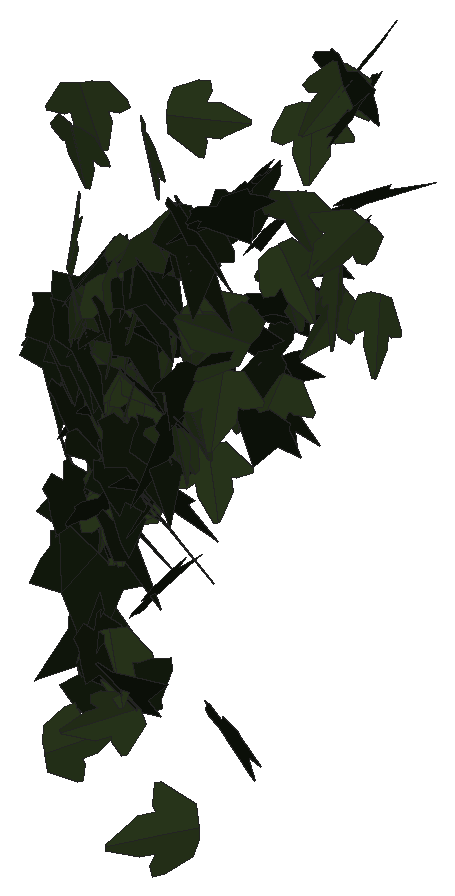
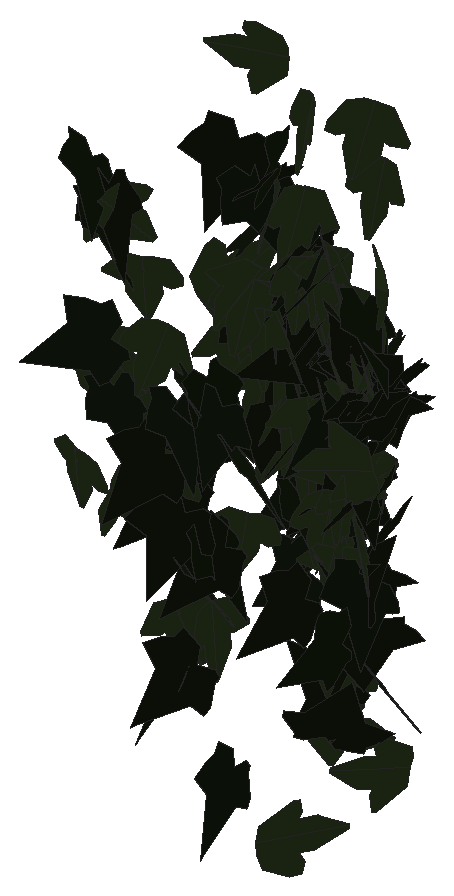
# SketchUp Ruby script. Lengths in inches.
U = 1.inch
M = Sketchup.active_model
def pt(a) = Geom::Point3d.new(a.map { |v| v * U })
def face(e, loops, mat)
  f = e.add_face(loops[0].map { |a| pt(a) })
  loops[1..].each { |l| e.add_face(l.map { |a| pt(a) }).erase! }
  f.material = f.back_material = mat if mat
  f
end
# faces: each face lists its corners as indices into pts; further lists are holes
def faces(e, pts, list, mat = nil) = list.each { |f| face(e, (f[0].is_a?(Array) ? f : [f]).map { |l| l.map { |i| pts[i] } }, mat) }
# xy, xz, yz: faces in a plane at the given z, y or x. An outline is a flat list of corners, or four numbers for a rectangle; further outlines are holes
def ring(l) = l.size == 4 ? [[l[0], l[1]], [l[2], l[1]], [l[2], l[3]], [l[0], l[3]]] : l.each_slice(2).to_a
def flat(e, list, mat, &to3) = list.each { |f| face(e, (f[0].is_a?(Array) ? f : [f]).map { |l| ring(l).map { |u, v| to3.(u, v) } }, mat) }
def xy(e, z, list, mat = nil) = flat(e, list, mat) { |x, y| [x, y, z] }
def xz(e, y, list, mat = nil) = flat(e, list, mat) { |x, z| [x, y, z] }
def yz(e, x, list, mat = nil) = flat(e, list, mat) { |y, z| [x, y, z] }
def lines(e, pts, list) = list.each { |a, b| e.add_line(pt(pts[a]), pt(pts[b])) }
# prism: a flat outline (further loops are holes) pulled along v
def prism(e, loops, v, mat = nil)
  f = face(e, loops, mat); d = Geom::Vector3d.new(v.map { |x| x * U })
  f.pushpull(f.normal.samedirection?(d) ? d.length : -d.length)
end
def box(e, o, s, mat = nil) = prism(e, [[o, [o[0] + s[0], o[1], o[2]], [o[0] + s[0], o[1] + s[1], o[2]], [o[0], o[1] + s[1], o[2]]]], [0, 0, s[2]], mat)
def at(x, y, z, deg = 0) = Geom::Transformation.translation(pt([x, y, z])) * Geom::Transformation.rotation(ORIGIN, Z_AXIS, deg.degrees)
def axes(o, x, y, z) = Geom::Transformation.new([*x, 0, *y, 0, *z, 0, *pt(o).to_a, 1])
def part(name) = M.definitions.add(name)
# library, detail: a bought-in or finely detailed component or shape, given as its bounding box
def library(name, o, s) = part(name).tap { |d| box(d.entities, o, s) }
def detail(e, o, s) = box(e.add_group.entities, o, s)
def put(e, d, t, mat = nil) = e.add_instance(d, t).tap { |i| i.material = mat if mat }
def group(e, t, mat = nil) = e.add_group.tap { |g| g.transformation = t; g.material = mat if mat }.entities
root = M.entities
M.materials.add("efeu1").color = [18, 25, 13]
M.materials.add("efeu2").color = [43, 57, 29]
c1 = part("ivyleaf_10")
p = [[0,0.5,-0.03],[-0.0625,2.02,-0.43],[-0.19,2.01,-0.46],[-0.54,1.05,-0.29],[-0.52,0.625,-0.18],[-0.83,0.76,-0.28],
  [-1.16,0.64,-0.33],[-1.15,0.33,-0.24],[-0.77,-0.39,0.02],[-0.3,-0.51,0.16],[0.04,-0.48,0.23],[-0.02,2.01,-0.4375],
  [-0.06,2.01,-0.43],[0.04,-0.49,0.23],[0.67,-0.49,0.14],[1.38,0.36,-0.2],[1.375,0.51,-0.24],[0.81,0.65,-0.19],
  [0.62,0.59,-0.15],[0.6,1.09,-0.28],[0.5,1.23,-0.31]]
faces(c1.entities,p,[[0,1,2,3,4,5,6,7,8,9,10],[11,12,0,13,14,15,16,17,18,19,20]],"efeu2")
c2 = part("ivyleaf_9")
p = [[1.54,2.16,1.25],[1.36,2.04,1.19],[-0.21,0.99,0.68],[-0.71,1.11,0.82],[-0.85,0.86,0.67],[-0.8,0.17,0.21],
  [-0.9,-0.01,0.1],[-0.67,-0.16,-0.02],[-0.08,-0.08,-0.05],[-0.03,-0.6,-0.4],[0.65,-0.88,-0.66],[0.83,-0.6,-0.49],
  [1.29,-0.42,-0.43],[1.8125,-0.07,-0.26],[1.21,0.44,0.15]]
faces(c2.entities,p,[[0,1,2,3,4,5,6,7,8,9,10,11,12,13,14]],"efeu1")
put(root,c1,axes([562.63,132.48,226.13],[0.74487,-0.56647,-0.14982],[-0.10251,0.1126,-0.9354],[0.57691,0.7514,0.02723]))
put(root,c2,axes([565.32,132.36,223.59],[0.01883,0.78936,-0.47762],[0.0076,-0.47783,-0.78941],[-0.92257,0.01218,-0.01626]))
put(root,c2,axes([560.59,132.81,223.19],[0.44309,-0.86355,0.20883],[0.08663,-0.19025,-0.97055],[0.88421,0.45138,-0.00955]))
put(root,c2,axes([562.13,131.96,218.41],[0.19063,0.88377,0.03705],[0.00683,0.03643,-0.9041],[-0.88452,0.19075,0.001]))
put(root,c2,axes([564.68,132.45,228.39],[0.75441,-0.54746,-0.08485],[-0.06586,0.0537,-0.9321],[0.55007,0.75726,0.00476]))
put(root,c1,axes([563.63,132.29,230.39],[-0.73079,0.6038,0.11548],[-0.12463,0.03014,-0.94632],[-0.60198,-0.73924,0.05574]))
put(root,c1,axes([564.97,132.28,231.75],[0.02233,-0.04625,-0.96103],[0.95551,0.11382,0.01673],[0.11285,-0.95453,0.04856]))
put(root,c1,axes([561.28,132.41,231.05],[-0.85143,-0.39436,-0.18271],[0.19871,0.0042,-0.93506],[0.38655,-0.8708,0.07823]))
put(root,c2,axes([560.5,132.39,221.16],[0.68747,-0.54835,-0.26594],[-0.17473,0.20672,-0.87793],[0.58385,0.70753,0.0504]))
put(root,c1,axes([562.29,132.86,211.09],[0.19129,0.23199,-0.85565],[-0.75388,-0.41804,-0.28188],[-0.4665,0.7707,0.10466]))
put(root,c2,axes([562.25,132.53,217.35],[0.65579,-0.65148,-0.14998],[-0.10696,0.10514,-0.92438],[0.6599,0.66446,-0.00079]))
put(root,c2,axes([562.71,132.72,224.01],[0.43622,-0.82316,-0.10756],[-0.05038,0.09504,-0.9316],[0.82863,0.43912,-0.00001]))
put(root,c2,axes([564.9,133.01,227.72],[-0.06625,-0.92627,0.03449],[-0.00824,-0.03399,-0.92862],[0.92687,-0.06651,-0.00579]))
put(root,c1,axes([560.69,131.97,209.86],[0.12519,0.06353,-0.9519],[0.65453,0.69275,0.13232],[0.69408,-0.66474,0.04691]))
put(root,c2,axes([560.49,132.45,218.1],[0.50144,-0.62284,-0.48454],[-0.28082,0.39567,-0.79921],[0.73746,0.57417,0.02513]))
put(root,c1,axes([562.64,132.87,224.18],[0.55748,-0.7265,0.19251],[0.17202,-0.10998,-0.91322],[0.73162,0.57944,0.06803]))
put(root,c2,axes([561.23,132.76,213.46],[-0.836,0.31556,-0.01671],[0.01566,-0.00583,-0.89357],[-0.31561,-0.83614,-0.00008]))
put(root,c2,axes([562.55,132.79,220.46],[0.34306,-0.83725,-0.24043],[0.00998,0.26216,-0.89869],[0.87103,0.32675,0.10499]))
put(root,c1,axes([563.72,132.41,227.34],[-0.31987,-0.85172,-0.44466],[0.15168,0.41801,-0.9098],[0.94876,-0.35399,-0.00446]))
put(root,c2,axes([561.92,132.73,211.86],[0.76255,0.26444,-0.41131],[0.38974,0.1315,0.8071],[0.29531,-0.85637,-0.00308]))
put(root,c2,axes([561.53,132.58,213.52],[0.43952,-0.62135,-0.47233],[-0.26511,0.39099,-0.76105],[0.73409,0.51323,0.00795]))
put(root,c2,axes([562.2,132.86,224.65],[-0.80671,0.38177,-0.19856],[0.16061,-0.12429,-0.89146],[-0.39923,-0.82143,0.0426]))
put(root,c2,axes([562.9,132.77,221.93],[0.71188,-0.4311,0.38388],[0.36398,-0.13784,-0.82976],[0.44803,0.79696,0.06414]))
put(root,c1,axes([565.95,133.41,224.26],[-0.39531,-0.4169,-0.95431],[-0.6168,-0.72872,0.57385],[-0.83909,0.73208,0.02776]))
put(root,c1,axes([562.65,132.31,225.79],[0.12954,0.80433,0.45266],[-0.1627,0.46984,-0.7883],[-0.90851,0.03055,0.20572]))
put(root,c1,axes([560.78,132.6,229.45],[-0.9317,0.17086,0.08642],[-0.08066,0.03915,-0.94694],[-0.17366,-0.93488,-0.02386]))
put(root,c2,axes([562,132.43,219.26],[0.68634,-0.3354,-0.48287],[-0.31174,0.4217,-0.73601],[0.49847,0.72554,0.20457]))
put(root,c2,axes([563.51,132.66,218.25],[0.87916,-0.33856,-0.02252],[-0.02247,0.00433,-0.94208],[0.33856,0.87943,-0.00403]))
put(root,c1,axes([560.85,132.63,224.12],[-0.7452,0.5426,-0.01916],[0.0167,-0.00962,-0.92181],[-0.54268,-0.74538,-0.00205]))
put(root,c1,axes([562.1,132.62,224.96],[0.69837,0.56841,0.20975],[0.03916,0.27705,-0.8812],[-0.60461,0.67451,0.1852]))
put(root,c2,axes([559.94,133.29,222.18],[-0.13117,-0.9069,0.01351],[0.00328,-0.01413,-0.91633],[0.907,-0.13111,0.00527]))
put(root,c1,axes([561.84,132.79,213.18],[0.7834,0.35112,0.25277],[0.22312,0.12006,-0.8583],[-0.37066,0.81436,0.01756]))
put(root,c2,axes([559.83,133.1875,223.13],[0.1269,-0.91044,-0.05985],[-0.01578,0.05823,-0.91921],[0.91227,0.12765,-0.00757]))
put(root,c2,axes([563.16,132.625,226.17],[0.81229,-0.27945,-0.33574],[-0.30267,0.15106,-0.85802],[0.31496,0.86586,0.04134]))
put(root,c2,axes([562.63,133.01,225.45],[0.3718,-0.83673,-0.16505],[0.01002,0.18433,-0.91188],[0.8528,0.36263,0.08267]))
put(root,c1,axes([561.98,132.81,217.83],[0.65456,0.6089,0.12715],[0.10691,0.0717,-0.89375],[-0.61277,0.66292,-0.02012]))
put(root,c2,axes([563.3,133.31,220.14],[0.21438,-0.87178,0.1773],[0.00863,-0.18033,-0.89711],[0.88959,0.21183,-0.03402]))
put(root,c2,axes([563.25,132.8,226.15],[0.28214,-0.73153,-0.50728],[-0.18415,0.47268,-0.78405],[0.87095,0.33692,-0.00145]))
put(root,c1,axes([560.62,132.81,223.65],[-0.29086,0.87086,-0.01631],[-0.10038,-0.0506,-0.91139],[-0.86521,-0.28689,0.11122]))
put(root,c1,axes([560.84,133.09,223.69],[0.46679,-0.78576,0.08376],[0.04543,-0.07043,-0.91395],[0.7889,0.46899,0.00308]))
put(root,c1,axes([564.48,132.8,227.41],[-0.52438,0.7715,-0.06941],[0.04242,-0.05509,-0.93283],[-0.77345,-0.52608,-0.0041]))
put(root,c2,axes([564.48,133.07,226.88],[0.52412,-0.76443,-0.03084],[0.06021,0.07848,-0.92208],[0.76268,0.51913,0.09399]))
put(root,c2,axes([561.9,132.98,224.17],[0.55785,-0.69879,-0.16171],[-0.02824,0.1833,-0.88952],[0.7167,0.55113,0.09081]))
put(root,c1,axes([561.6,132.75,222.25],[0.42938,-0.03804,0.80607],[0.73946,0.38414,-0.37576],[-0.32311,0.82859,0.21121]))
put(root,c1,axes([561,133.11,223.71],[0.26037,-0.88612,0.04843],[0.02003,-0.04459,-0.92355],[0.88721,0.26105,0.00664]))
put(root,c1,axes([560.68,132.54,225.63],[0.39334,-0.38137,0.77451],[-0.56516,0.52963,0.54781],[-0.65261,-0.68852,-0.0076]))
put(root,c2,axes([565.09,132.96,227.91],[-0.2305,0.8001,-0.41493],[-0.01064,-0.43067,-0.82454],[-0.90123,-0.19955,0.11586]))
put(root,c1,axes([565.66,133.05,222.78],[0.5315,0.74323,-0.16148],[-0.13147,-0.10426,-0.91258],[-0.74912,0.54561,0.04558]))
put(root,c2,axes([560.24,133.41,222.51],[-0.508,-0.73449,-0.17827],[0.10901,0.14135,-0.893],[0.74791,-0.51948,0.00907]))
put(root,c1,axes([561.7,133.45,223.6],[0.49749,-0.62812,0.43089],[0.26077,-0.34311,-0.80123],[0.71568,0.56164,-0.00758]))
put(root,c1,axes([563.52,133.81,207.29],[-0.16835,0.13796,1.07578],[-0.2837,-1.05636,0.09107],[1.04683,-0.2641,0.19768]))
put(root,c2,axes([564,133.61,221.28],[-0.37612,0.37539,-0.96435],[0.55373,-0.79381,-0.52497],[-0.87423,-0.6643,0.08237]))
put(root,c1,axes([562.45,133.1,222.03],[0.50725,-0.73779,-0.19012],[-0.07471,0.17914,-0.89449],[0.75822,0.51123,0.03905]))
put(root,c1,axes([563.57,133.27,223.14],[0.65651,-0.63349,0.00392],[0.0005,-0.00513,-0.91231],[0.6335,0.6565,-0.00334]))
put(root,c2,axes([561.4,133.45,223.3],[-0.6803,-0.41985,-0.43111],[0.41112,0.15088,-0.79571],[0.43944,-0.79114,0.07703]))
put(root,c2,axes([560.68,133.4,222.66],[-0.13177,-0.86286,-0.26158],[0.01663,0.26199,-0.87258],[0.90148,-0.13095,-0.02214]))
put(root,c1,axes([563.05,133.1,225.87],[0.55558,0.72457,0.05902],[0.04704,0.03829,-0.91295],[-0.72545,0.55739,-0.014]))
put(root,c2,axes([562.04,133.5625,218.61],[-0.12828,-0.89547,-0.05421],[0.00188,0.0545,-0.90459],[0.8971,-0.12816,-0.00585]))
put(root,c2,axes([561.09,132.83,225.09],[-0.36312,0.85796,0.0877],[-0.02253,0.08569,-0.93156],[-0.86214,-0.3636,-0.01259]))
put(root,c1,axes([561.39,133.26,222.2],[0.89313,-0.04927,0.11951],[0.12182,0.04166,-0.8932],[0.04324,0.90012,0.04788]))
put(root,c2,axes([560.6,133.63,216.96],[-0.63249,-0.62089,-0.15637],[0.15777,0.0619,-0.8839],[0.62054,-0.64859,0.06534]))
put(root,c2,axes([560.3,133.36,219.46],[0.63148,-0.53306,0.33993],[0.30488,-0.16414,-0.82376],[0.55385,0.69813,0.06588]))
put(root,c1,axes([563.125,133.15,225.79],[-0.37959,-0.81563,-0.17559],[0.07036,0.16093,-0.89963],[0.83135,-0.38603,-0.00403]))
put(root,c2,axes([563.49,132.48,215.45],[0.32722,0.45031,0.71547],[0.16499,0.71842,-0.52763],[-0.82913,0.32068,0.17737]))
put(root,c2,axes([565.81,132.75,228.81],[0.48083,0.79451,-0.01834],[-0.0089,-0.01606,-0.92868],[-0.79467,0.48091,-0.0007]))
put(root,c1,axes([564.51,133.15,221.78],[-0.90261,0.17243,-0.09131],[0.09237,-0.00303,-0.91882],[-0.17186,-0.90721,-0.01429]))
put(root,c1,axes([561.26,133.55,217.78],[-0.18047,0.75935,-0.45575],[-0.02238,-0.46888,-0.77236],[-0.88534,-0.14294,0.11243]))
put(root,c1,axes([563.96,133.23,220.97],[-0.36272,0.84209,-0.06263],[-0.00842,-0.07177,-0.91618],[-0.84438,-0.36102,0.03604]))
put(root,c2,axes([562.55,132.81,223.15],[0.63352,0.26515,0.61168],[0.54189,0.28673,-0.68553],[-0.38835,0.83264,0.04128]))
put(root,c2,axes([560.79,133.56,222.43],[0.42025,-0.79543,-0.09642],[0.00271,0.1103,-0.89803],[0.80125,0.41683,0.05362]))
put(root,c2,axes([563.2,133.15,218.32],[-0.44926,0.78437,0.09153],[-0.03687,0.08436,-0.90386],[-0.78883,-0.45066,-0.00988]))
put(root,c1,axes([563.68,133.25,220.63],[-0.55745,-0.6346,-0.35867],[0.25215,0.25578,-0.84445],[0.68394,-0.61153,0.01899]))
put(root,c2,axes([560.64,133.75,219.41],[0.18741,-0.87156,-0.08214],[-0.00461,0.08302,-0.89138],[0.8754,0.18702,0.01289]))
put(root,c2,axes([560.95,133.24,220.4375],[-0.10282,0.86544,-0.20515],[0.04891,-0.2007,-0.87119],[-0.88808,-0.11125,-0.02423]))
put(root,c2,axes([560.4,133.82,215.18],[-0.40979,-0.92763,-0.36512],[0.14375,0.33565,-1.01411],[0.98648,-0.43426,-0.0039]))
put(root,c1,axes([562.91,133.36,219.93],[-0.80664,0.27027,0.33586],[-0.34932,0.00779,-0.84524],[-0.25263,-0.87373,0.09635]))
put(root,c1,axes([564.86,133.43,224.45],[-0.90078,-0.15961,-0.07893],[0.07626,0.022,-0.91477],[0.1609,-0.90396,-0.00832]))
put(root,c2,axes([560.68,133.29,223.2],[-0.65591,0.08888,0.63468],[0.62863,-0.08744,0.6619],[0.12467,0.90851,0.00162]))
put(root,c1,axes([564.91,133.17,224.86],[0.39814,0.64141,0.53402],[0.20576,0.49797,-0.75152],[-0.80885,0.4424,0.07168]))
put(root,c1,axes([562.53,133.56,221.65],[0.56989,0.70089,-0.06359],[-0.10941,0.0074,-0.89891],[-0.69521,0.57338,0.08934]))
put(root,c2,axes([560.86,133.45,216.09],[0.2359,-0.56937,0.88839],[-0.36834,0.80863,0.61605],[-0.98881,-0.43705,-0.01754]))
put(root,c1,axes([560.33,133.71,220.43],[0.33853,0.79194,-0.24251],[-0.14784,-0.19999,-0.85949],[-0.81494,0.36526,0.05519]))
put(root,c1,axes([561.77,133.61,218.72],[-0.64279,-0.61654,-0.1417],[0.17285,0.02316,-0.88486],[0.60855,-0.65782,0.10165]))
put(root,c2,axes([561.96,133.47,211.17],[-1.00694,-0.35404,0.19197],[0.1893,0.04022,1.06708],[-0.35547,1.02429,0.02446]))
put(root,c1,axes([561.34,133.6875,217.27],[0.79814,0.41228,0.0331],[0.03468,0.00498,-0.89826],[-0.41215,0.79881,-0.01148]))
put(root,c1,axes([564.22,133.6,223.75],[-0.86542,0.13442,0.26468],[-0.26837,-0.00554,-0.87466],[-0.1269,-0.90497,0.04467]))
put(root,c2,axes([561.29,133.28,221.8],[0.8587,0.27287,0.05516],[0.02512,0.1022,-0.89654],[-0.27726,0.85437,0.08963]))
put(root,c1,axes([560.92,133.8,219.76],[-0.35726,-0.81536,-0.11006],[0.24732,0.00801,-0.86217],[0.78471,-0.37374,0.22162]))
put(root,c2,axes([560.4375,133.67,216.8],[0.06057,0.89691,-0.00348],[0.00047,-0.00352,-0.89895],[-0.89691,0.06057,-0.00071]))
put(root,c1,axes([560.29,134.1,218.58],[0.56751,-0.65356,-0.19834],[-0.07913,0.19322,-0.86311],[0.67839,0.56927,0.06525]))
put(root,c1,axes([560.16,134.32,220.83],[0.23551,0.13556,1.03923],[0.94754,0.42759,-0.27051],[-0.44782,0.97603,-0.02583]))
put(root,c1,axes([563.24,135.49,218.5],[0.75224,0.46618,0.1884],[0.14136,0.12927,-0.88431],[-0.48253,0.76463,0.03464]))
put(root,c2,axes([559.875,135.53,215.73],[0.82995,-0.29876,0.07791],[0.07665,-0.0171,-0.88203],[0.29908,0.83342,0.00983]))
put(root,c2,axes([565.13,135.46,220.66],[0.57439,0.30633,-0.64526],[-0.57602,-0.29097,-0.65089],[-0.42237,0.8134,0.01017]))
put(root,c2,axes([563.84,135.43,210.2],[0.78738,0.04929,-0.48881],[-0.49029,0.02011,-0.78774],[-0.03125,0.92655,0.04311]))
put(root,c2,axes([561.09,135.7,216.84],[0.89053,0.04618,0.03504],[0.03465,0.00842,-0.8917],[-0.04647,0.89118,0.00661]))
put(root,c2,axes([562.62,137.95,219.88],[-0.05377,0.84026,0.33725],[-0.08972,0.33124,-0.83959],[-0.90096,-0.08313,0.06348]))
put(root,c1,axes([563.86,138.67,225.67],[-0.90436,-0.12101,-0.21653],[0.21696,0.01089,-0.91225],[0.12024,-0.92986,0.01749]))
put(root,c1,axes([565.1875,139.22,229.81],[0.46081,0.56196,-0.60234],[-0.44362,-0.41226,-0.72402],[-0.69413,0.63655,0.06284]))
put(root,c1,axes([565.51,139.32,225.04],[-0.48986,-0.49853,0.65295],[-0.36431,-0.54955,-0.69289],[0.73631,-0.60357,0.09157]))
put(root,c1,axes([563.25,138.91,223.47],[0.71265,0.1701,0.58473],[0.56638,0.14557,-0.73262],[-0.22374,0.91027,0.0079]))
put(root,c2,axes([565.96,138.86,229.48],[-0.492,0.7917,0.02654],[-0.02273,0.01711,-0.93206],[-0.79182,-0.49241,0.01027]))
put(root,c2,axes([561.68,139.15,225.26],[-0.42252,0.70772,-0.39931],[0.12563,-0.38777,-0.82018],[-0.80283,-0.43314,0.08181]))
put(root,c1,axes([564,139.19,228.2],[0.83723,0.40918,0.04116],[0.03645,0.01915,-0.93187],[-0.40963,0.83802,0.0012]))
put(root,c2,axes([562.375,139.31,225.11],[-0.76887,0.45023,-0.18621],[0.14024,-0.12864,-0.89013],[-0.4666,-0.78057,0.03929]))
put(root,c2,axes([565.41,139.07,230.24],[0.50915,0.1908,-0.77146],[-0.71591,-0.28762,-0.54362],[-0.345,0.87844,-0.01043]))
put(root,c1,axes([564.59,139.54,222.99],[0.69944,-0.48932,0.40341],[0.36857,-0.17509,-0.85141],[0.51608,0.78822,0.06131]))
put(root,c2,axes([561.45,139.4,220.43],[-0.47015,0.7237,-0.34333],[0.20648,-0.27515,-0.86274],[-0.77394,-0.51304,-0.02161]))
put(root,c2,axes([560.6,139.36,223.48],[-0.70679,0.55722,0.10387],[-0.07347,0.07455,-0.89993],[-0.56203,-0.71048,-0.01297]))
put(root,c2,axes([566.11,138.95,230.84],[-0.14615,0.84499,0.38648],[-0.06444,0.38107,-0.85753],[-0.92694,-0.15972,-0.00132]))
put(root,c2,axes([562.45,139.67,219.75],[-0.75251,0.53567,0.06161],[-0.07213,0.00482,-0.92292],[-0.53435,-0.75501,0.03782]))
put(root,c2,axes([562.56,139.5,224.32],[-0.21748,0.8807,-0.01749],[-0.00305,-0.01876,-0.90712],[-0.88087,-0.21737,0.00746]))
put(root,c1,axes([562.64,139.72,222.35],[-0.90262,-0.00996,-0.06789],[0.06778,0.00991,-0.90263],[0.01067,-0.90511,-0.00914]))
put(root,c2,axes([560.91,139.56,220.25],[0.90367,0.21326,-0.00118],[0.00487,-0.02576,-0.92812],[-0.21321,0.9033,-0.02619]))
put(root,c2,axes([562.34,139.41,221.83],[0.78703,0.45811,0.21935],[0.19005,0.10952,-0.91065],[-0.47101,0.80965,-0.00093]))
put(root,c2,axes([564.66,139.7,224.22],[-0.28209,0.86545,-0.09653],[-0.07092,-0.12396,-0.90415],[-0.86792,-0.27115,0.10525]))
put(root,c1,axes([560.84,139.98,218.22],[-0.07215,-0.91445,-0.08181],[0.04868,0.07814,-0.91632],[0.91681,-0.07611,0.04222]))
put(root,c2,axes([561.12,139.34,224.63],[0.1508,0.86465,0.2661],[-0.05925,0.27864,-0.87179],[-0.90273,0.12615,0.10167]))
put(root,c1,axes([563.89,140.61,221.53],[0.05479,0.54628,-0.75963],[-0.23578,-0.72832,-0.54077],[-0.90547,0.2227,0.09485]))
put(root,c1,axes([565.44,140.36,221.98],[0.89013,-0.19193,0.23887],[0.23608,-0.03826,-0.91051],[0.19534,0.92083,0.01195]))
put(root,c1,axes([561.89,140.26,218.25],[0.66472,0.56842,-0.29043],[-0.34864,-0.02793,-0.85263],[-0.53469,0.72486,0.19489]))
put(root,c2,axes([565.04,139.58,225.67],[0.70741,0.2423,0.59218],[0.3373,0.60895,-0.65209],[-0.5437,0.69303,0.36594]))
put(root,c2,axes([561.92,140.07,221.21],[0.54022,0.7173,-0.01855],[-0.01047,-0.01533,-0.89797],[-0.71746,0.54032,-0.00086]))
put(root,c2,axes([562.7,140.03,222.9],[0.58627,0.6395,0.26381],[0.17831,0.19442,-0.86757],[-0.6684,0.61279,-0.00006]))
put(root,c2,axes([561,141.28,217.29],[0.70751,-0.15041,-0.56051],[-0.48599,0.3295,-0.70186],[0.31719,0.84034,0.17488]))
put(root,c2,axes([560.29,141.59,217.53],[0.48988,0.63225,0.44227],[0.23092,0.37974,-0.79862],[-0.73622,0.5398,0.04379]))
